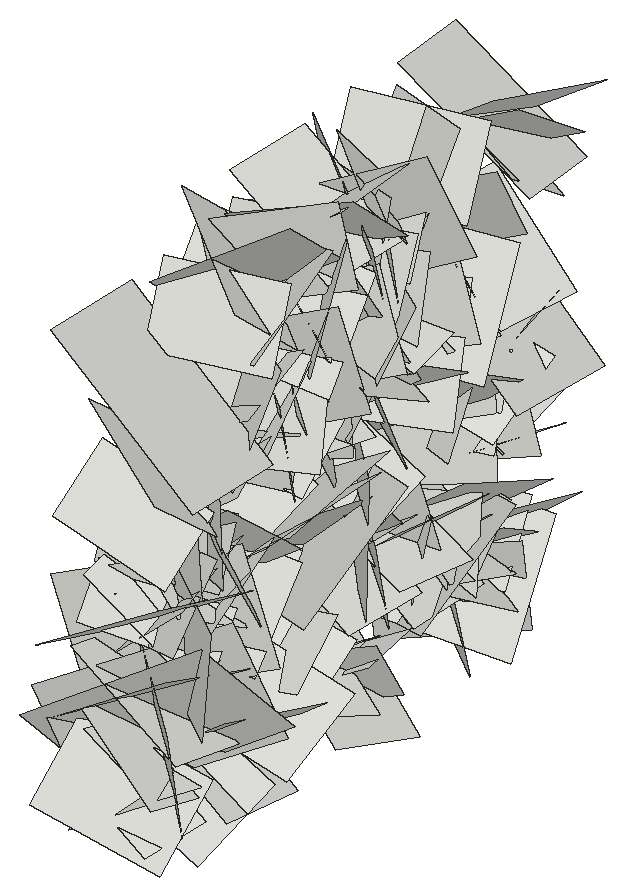
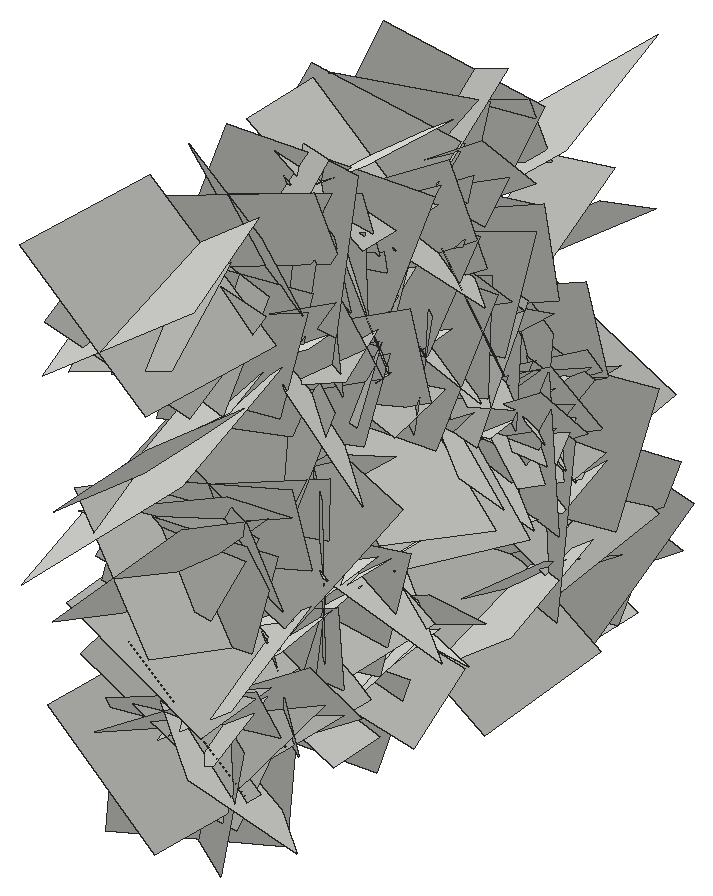
# SketchUp Ruby script. Lengths in inches.
U = 1.inch
M = Sketchup.active_model
def pt(a) = Geom::Point3d.new(a.map { |v| v * U })
def face(e, loops, mat)
  f = e.add_face(loops[0].map { |a| pt(a) })
  loops[1..].each { |l| e.add_face(l.map { |a| pt(a) }).erase! }
  f.material = f.back_material = mat if mat
  f
end
# faces: each face lists its corners as indices into pts; further lists are holes
def faces(e, pts, list, mat = nil) = list.each { |f| face(e, (f[0].is_a?(Array) ? f : [f]).map { |l| l.map { |i| pts[i] } }, mat) }
# xy, xz, yz: faces in a plane at the given z, y or x. An outline is a flat list of corners, or four numbers for a rectangle; further outlines are holes
def ring(l) = l.size == 4 ? [[l[0], l[1]], [l[2], l[1]], [l[2], l[3]], [l[0], l[3]]] : l.each_slice(2).to_a
def flat(e, list, mat, &to3) = list.each { |f| face(e, (f[0].is_a?(Array) ? f : [f]).map { |l| ring(l).map { |u, v| to3.(u, v) } }, mat) }
def xy(e, z, list, mat = nil) = flat(e, list, mat) { |x, y| [x, y, z] }
def xz(e, y, list, mat = nil) = flat(e, list, mat) { |x, z| [x, y, z] }
def yz(e, x, list, mat = nil) = flat(e, list, mat) { |y, z| [x, y, z] }
def lines(e, pts, list) = list.each { |a, b| e.add_line(pt(pts[a]), pt(pts[b])) }
# prism: a flat outline (further loops are holes) pulled along v
def prism(e, loops, v, mat = nil)
  f = face(e, loops, mat); d = Geom::Vector3d.new(v.map { |x| x * U })
  f.pushpull(f.normal.samedirection?(d) ? d.length : -d.length)
end
def box(e, o, s, mat = nil) = prism(e, [[o, [o[0] + s[0], o[1], o[2]], [o[0] + s[0], o[1] + s[1], o[2]], [o[0], o[1] + s[1], o[2]]]], [0, 0, s[2]], mat)
def at(x, y, z, deg = 0) = Geom::Transformation.translation(pt([x, y, z])) * Geom::Transformation.rotation(ORIGIN, Z_AXIS, deg.degrees)
def axes(o, x, y, z) = Geom::Transformation.new([*x, 0, *y, 0, *z, 0, *pt(o).to_a, 1])
def part(name) = M.definitions.add(name)
# library, detail: a bought-in or finely detailed component or shape, given as its bounding box
def library(name, o, s) = part(name).tap { |d| box(d.entities, o, s) }
def detail(e, o, s) = box(e.add_group.entities, o, s)
def put(e, d, t, mat = nil) = e.add_instance(d, t).tap { |i| i.material = mat if mat }
def group(e, t, mat = nil) = e.add_group.tap { |g| g.transformation = t; g.material = mat if mat }.entities
root = M.entities
c1 = part("Component\#6")
p = [[0.01,0,0],[0,3.24,4.54],[4.32,3.24,4.54],[4.33,0,0]]
faces(c1.entities,p,[[0,1,2,3]])
put(root,c1,axes([400.91,169.05,21.98],[0.04882,0.58162,0.59704],[-0.02934,0.59868,-0.58109],[0.88303,-0.01226,-0.05232]))
put(root,c1,axes([404.88,173.67,32.24],[0.05341,-0.65994,-0.37026],[0.06447,-0.36634,0.66124],[-0.79951,-0.07362,0.02859]))
put(root,c1,axes([404.88,173.11,21.9],[0.05319,-0.68826,0.19248],[0.04456,0.19546,0.68797],[-0.75624,-0.03689,0.05408]))
put(root,c1,axes([400.91,173.29,20.87],[0.09428,-0.62013,-0.08152],[0.03551,-0.0775,0.6261],[0.66205,0.09247,-0.02197]))
put(root,c1,axes([404.88,173.29,20.87],[-0.09428,-0.62013,-0.08152],[-0.03551,-0.0775,0.6261],[-0.66205,0.09247,-0.02197]))
put(root,c1,axes([404.88,173.15,22.23],[-0.01199,-0.5915,0.12784],[-0.10227,0.12799,0.58366],[-0.63327,-0.00947,-0.09668]))
put(root,c1,axes([400.91,174.01,26.46],[-0.07872,-0.97306,0.24072],[0.0738,0.23579,0.97461],[1.05998,-0.08868,-0.04998]))
put(root,c1,axes([400.91,172.13,35.78],[0.07615,0.65901,-0.5201],[0.04859,-0.52431,-0.658],[0.88857,-0.02781,0.08055]))
put(root,c1,axes([400.91,173.5,20.5],[-0.29119,-0.77592,0.90535],[0.00734,0.92801,0.79744],[1.26387,-0.18415,0.20396]))
put(root,c1,axes([404.88,171.18,26.98],[0.09963,0.88743,-0.23237],[-0.05305,-0.22828,-0.89204],[-0.97094,0.10354,0.02489]))
put(root,c1,axes([400.91,171.18,26.98],[-0.09963,0.88743,-0.23237],[0.05305,-0.22828,-0.89204],[0.97094,0.10354,0.02489]))
put(root,c1,axes([400.91,170.16,39.2],[-0.24703,1.2789,-0.21613],[-0.13589,-0.24123,-1.28918],[1.36812,0.20696,-0.16707]))
put(root,c1,axes([404.88,172,20.82],[0.19013,-0.4174,1.11707],[0.18593,1.12659,0.39279],[-1.25031,0.10406,0.22828]))
put(root,c1,axes([400.91,172,20.82],[-0.19013,-0.4174,1.11707],[-0.18593,1.12659,0.39279],[1.25031,0.10406,0.22828]))
put(root,c1,axes([400.91,171.52,27.71],[-0.03995,0.48298,0.66079],[-0.01207,0.66111,-0.48387],[0.8675,0.03144,0.0237]))
put(root,c1,axes([404.88,171.52,27.71],[0.03995,0.48298,0.66079],[0.01207,0.66111,-0.48387],[-0.8675,0.03144,0.0237]))
put(root,c1,axes([400.91,171.36,22.89],[0.02535,0.88672,0.32576],[-0.06435,0.32663,-0.88464],[0.99927,-0.00146,-0.06523]))
put(root,c1,axes([404.88,175.14,30.45],[0.22771,0.17317,-1.07869],[-0.0194,-1.09862,-0.18001],[-1.15789,0.05246,-0.20912]))
put(root,c1,axes([400.91,175.14,30.45],[-0.22771,0.17317,-1.07869],[0.0194,-1.09862,-0.18001],[1.15789,0.05246,-0.20912]))
put(root,c1,axes([404.88,174.95,31.63],[-0.12097,-0.07785,-0.70642],[-0.09105,-0.70871,0.09198],[-0.74781,0.09888,0.10307]))
put(root,c1,axes([400.91,174.95,31.63],[0.12097,-0.07785,-0.70642],[0.09105,-0.70871,0.09198],[0.74781,0.09888,0.10307]))
put(root,c1,axes([404.88,176.52,27.27],[-0.06139,-0.83333,-0.30669],[0.14477,-0.31205,0.82208],[-0.93005,0.00643,0.1482]))
put(root,c1,axes([400.91,176.52,27.27],[0.06139,-0.83333,-0.30669],[-0.14477,-0.31205,0.82208],[0.93005,0.00643,0.1482]))
put(root,c1,axes([404.88,174.16,29.86],[-0.19319,0.59277,-0.26834],[-0.07097,-0.29428,-0.60458],[-0.68606,-0.13648,0.1381]))
put(root,c1,axes([400.91,174.16,29.86],[0.19319,0.59277,-0.26834],[0.07097,-0.29428,-0.60458],[0.68606,-0.13648,0.1381]))
put(root,c1,axes([400.91,176.41,32.2],[0.11408,-0.0942,-0.79779],[0.0272,-0.8041,0.09841],[0.85109,0.03832,0.10379]))
put(root,c1,axes([400.91,172.625,27.43],[-0.01975,0.58315,0.74345],[0.01761,0.74368,-0.58292],[1.00141,-0.00157,0.02491]))
put(root,c1,axes([404.88,174.375,32.02],[0.18574,0.64681,-0.5499],[0.00393,-0.56207,-0.65994],[-0.8999,0.13105,-0.11638]))
put(root,c1,axes([400.91,176.05,33.17],[0.01986,0.50916,-0.88553],[-0.06176,-0.8837,-0.50934],[1.08099,-0.05984,-0.01283]))
put(root,c1,axes([404.88,178.05,19.9375],[0.14578,-1.0409,0.22357],[0.02192,0.228,1.04879],[-1.1283,-0.13006,0.04926]))
put(root,c1,axes([400.91,178.05,19.9375],[-0.14578,-1.0409,0.22357],[-0.02192,0.228,1.04879],[1.1283,-0.13006,0.04926]))
put(root,c1,axes([404.88,177.7,39.03],[0.08239,-0.33737,-0.64844],[-0.10668,-0.65083,0.32654],[-0.76743,0.05425,-0.11501]))
put(root,c1,axes([400.91,173.36,27.66],[-0.12062,0.63946,0.63128],[-0.06443,0.62939,-0.6485],[0.9503,0.12384,0.03616]))
put(root,c1,axes([404.88,173.36,27.66],[0.12062,0.63946,0.63128],[0.06443,0.62939,-0.6485],[-0.9503,0.12384,0.03616]))
put(root,c1,axes([404.88,174.875,32.24],[-0.12053,0.70886,0.38052],[0.08644,0.39248,-0.70676],[-0.84842,-0.06072,-0.12606]))
put(root,c1,axes([400.91,174.875,32.24],[0.12053,0.70886,0.38052],[-0.08644,0.39248,-0.70676],[0.84842,-0.06072,-0.12606]))
put(root,c1,axes([404.88,178.15,33.23],[-0.08938,-0.00525,-0.60269],[0.06829,-0.60515,-0.00374],[-0.63521,-0.06432,0.0844]))
put(root,c1,axes([404.88,174.67,32.54],[0.17055,0.3665,0.95024],[0.03456,0.95968,-0.37566],[-1.07902,0.08867,0.13816]))
put(root,c1,axes([400.91,174.67,32.54],[-0.17055,0.3665,0.95024],[-0.03456,0.95968,-0.37566],[1.07902,0.08867,0.13816]))
put(root,c1,axes([400.91,174.9,23.69],[-0.06803,0.90477,0.33383],[0.16872,0.33992,-0.89067],[1.00823,0.00417,0.17157]))
put(root,c1,axes([404.88,175.43,34.87],[0.0411,0.62613,0.35799],[0.03637,0.3565,-0.62724],[-0.76365,0.05068,-0.01061]))
put(root,c1,axes([404.88,178.01,36.42],[-0.04909,-0.68925,0.58112],[0.09024,0.57594,0.68989],[-0.95135,0.0902,0.03545]))
put(root,c1,axes([400.91,178.01,36.42],[0.04909,-0.68925,0.58112],[-0.09024,0.57594,0.68989],[0.95135,0.0902,0.03545]))
put(root,c1,axes([400.91,177.13,31.79],[-0.078,-0.30439,1.03044],[-0.07955,1.03178,0.29943],[1.13614,0.05135,0.09171]))
put(root,c1,axes([404.88,176.26,32.94],[-0.03084,0.60524,0.59943],[0.03406,0.60013,-0.60439],[-0.90231,0.00196,-0.0433]))
put(root,c1,axes([400.91,176.26,32.94],[0.03084,0.60524,0.59943],[-0.03406,0.60013,-0.60439],[0.90231,0.00196,-0.0433]))
put(root,c1,axes([400.91,182.1,27.04],[-0.18817,-1.1788,-0.21223],[-0.10509,-0.19936,1.19019],[1.26526,-0.19187,0.06729]))
put(root,c1,axes([400.91,175.72,36.8],[-0.15665,0.75943,0.7145],[-0.11122,0.70715,-0.77331],[1.09966,0.17971,0.02357]))
put(root,c1,axes([404.88,175.72,36.8],[0.15665,0.75943,0.7145],[0.11122,0.70715,-0.77331],[-1.09966,0.17971,0.02357]))
put(root,c1,axes([404.88,180.11,41],[0.0874,0.13713,-0.78202],[0.02965,-0.78624,-0.13492],[-0.84107,-0.01347,-0.08602]))
put(root,c1,axes([404.88,177.89,30.77],[-0.05678,-0.11721,0.8526],[0.09083,0.84928,0.12214],[-0.90772,0.09231,-0.04111]))
put(root,c1,axes([400.91,177.89,30.77],[0.05678,-0.11721,0.8526],[-0.09083,0.84928,0.12214],[0.90772,0.09231,-0.04111]))
put(root,c1,axes([404.88,177.99,23.55],[-0.04107,0.5427,0.4395],[-0.20397,0.41484,-0.52921],[-0.71159,-0.15024,0.12632]))
put(root,c1,axes([400.91,177.99,23.55],[0.04107,0.5427,0.4395],[0.20397,0.41484,-0.52921],[0.71159,-0.15024,0.12632]))
put(root,c1,axes([400.91,182.77,28.15],[-0.11013,-1.0722,-0.31704],[-0.03816,-0.31503,1.07721],[1.18456,-0.10983,0.00522]))
put(root,c1,axes([400.91,180.66,33.34],[-0.08177,-0.45253,0.73357],[0.03972,0.73405,0.45677],[0.91278,-0.07248,0.04584]))
put(root,c1,axes([404.88,180.66,33.34],[0.08177,-0.45253,0.73357],[-0.03972,0.73405,0.45677],[-0.91278,-0.07248,0.04584]))
put(root,c1,axes([404.88,182.27,37.76],[0.22679,0.05489,-0.89691],[0.06736,-0.9206,-0.04118],[-0.95012,-0.05216,-0.217]))
put(root,c1,axes([404.88,182.09,31.375],[-0.0562,-0.72005,0.10613],[-0.07977,0.11126,0.71729],[-0.76737,0.04117,-0.08234]))
put(root,c1,axes([400.91,182.09,31.375],[0.0562,-0.72005,0.10613],[0.07977,0.11126,0.71729],[0.76737,0.04117,-0.08234]))
put(root,c1,axes([404.88,180.04,24.28],[-0.15161,0.71603,-0.23582],[-0.04269,-0.24694,-0.72538],[-0.79796,-0.12284,0.08362]))
put(root,c1,axes([400.91,180.04,24.28],[0.15161,0.71603,-0.23582],[0.04269,-0.24694,-0.72538],[0.79796,-0.12284,0.08362]))
put(root,c1,axes([400.91,181.67,36.78],[-0.05967,0.56874,-0.94691],[-0.29528,-0.9248,-0.5389],[1.13301,-0.21107,-0.19031]))
put(root,c1,axes([404.88,181.67,36.78],[0.05967,0.56874,-0.94691],[0.29528,-0.9248,-0.5389],[-1.13301,-0.21107,-0.19031]))
put(root,c1,axes([400.91,181.8125,37.17],[-0.0246,-0.63961,0.56311],[0.17949,0.54862,0.63013],[0.88529,-0.129,-0.11211]))
put(root,c1,axes([404.88,184.3,37.98],[0.01849,-0.42221,-1.00939],[0.24573,-0.98518,0.41609],[-1.13346,-0.22047,0.07374]))
put(root,c1,axes([400.91,184.3,37.98],[-0.01849,-0.42221,-1.00939],[-0.24573,-0.98518,0.41609],[1.13346,-0.22047,0.07374]))
put(root,c1,axes([400.91,185.38,28.27],[-0.28552,-0.8956,-0.93898],[-0.07116,-0.9481,0.92355],[1.37362,-0.23528,-0.14733]))
put(root,c1,axes([404.88,183.5625,38.07],[-0.03427,-0.86867,-0.02883],[0.01016,-0.0292,0.8692],[-0.92124,0.03199,0.01066]))
put(root,c1,axes([400.91,183.5625,38.07],[0.03427,-0.86867,-0.02883],[-0.01016,-0.0292,0.8692],[0.92124,0.03199,0.01066]))
put(root,c1,axes([404.88,181.88,29.24],[-0.0732,0.47057,-0.46808],[0.06498,-0.46407,-0.47558],[-0.70054,-0.09222,0.00479]))
put(root,c1,axes([400.91,180.55,24.45],[0.04702,0.95483,-0.28451],[-0.08229,-0.28062,-0.95386],[1.05288,-0.06457,-0.06184]))
put(root,c1,axes([404.88,182.11,23.57],[0.01533,0.32032,-0.55846],[-0.07998,-0.55391,-0.31966],[-0.67773,0.07262,0.02509]))
put(root,c1,axes([404.88,180.54,27.52],[-0.00647,0.86334,-0.00303],[0.00368,-0.003,-0.86336],[-0.91514,-0.00612,-0.00345]))
put(root,c1,axes([400.91,180.54,27.52],[0.00647,0.86334,-0.00303],[-0.00368,-0.003,-0.86336],[0.91514,-0.00612,-0.00345]))
put(root,c1,axes([400.91,181.12,36.49],[-0.0887,0.85058,-0.45713],[0.14057,-0.44437,-0.85112],[1.01388,0.13603,0.07801]))
put(root,c1,axes([404.88,184.65,28.76],[-0.04824,-0.62434,-0.28052],[0.09786,-0.28417,0.61748],[-0.7189,0.00321,0.10288]))
put(root,c1,axes([400.91,185.4,30.76],[-0.02152,-0.00963,-1.2106],[-0.23963,-1.18945,0.01326],[1.26071,-0.22625,-0.01814]))
put(root,c1,axes([404.88,181.75,22.9],[-0.07496,0.59984,0.04506],[-0.05269,0.03939,-0.60235],[-0.63545,-0.07402,0.04463]))
put(root,c1,axes([400.91,184.92,37.05],[0.01613,-0.13323,-0.78421],[0.01491,-0.78419,0.1335],[0.84304,0.01642,0.01265]))
put(root,c1,axes([404.88,184.92,37.05],[-0.01613,-0.13323,-0.78421],[-0.01491,-0.78419,0.1335],[-0.84304,0.01642,0.01265]))
put(root,c1,axes([404.88,182.91,34.72],[0.14912,-0.41506,0.98502],[0.044,0.99488,0.41329],[-1.13217,-0.016,0.1458]))
put(root,c1,axes([400.91,182.91,34.72],[-0.14912,-0.41506,0.98502],[-0.044,0.99488,0.41329],[1.13217,-0.016,0.1458]))
put(root,c1,axes([400.91,184.84,39.1],[0.02023,-0.20369,-0.6632],[0.11732,-0.65406,0.20407],[0.72599,0.11137,-0.0145]))
put(root,c1,axes([404.88,184.84,39.1],[-0.02023,-0.20369,-0.6632],[-0.11732,-0.65406,0.20407],[-0.72599,0.11137,-0.0145]))
put(root,c1,axes([400.91,182.78,23.92],[-0.06221,-0.24398,0.83625],[-0.07047,0.83695,0.23952],[0.92069,0.04758,0.07484]))
put(root,c1,axes([404.88,182.78,23.92],[0.06221,-0.24398,0.83625],[0.07047,0.83695,0.23952],[-0.92069,0.04758,0.07484]))
put(root,c1,axes([400.91,184.8,33.37],[0.19651,0.19461,-0.78555],[-0.01158,-0.80522,-0.20206],[0.85778,-0.05545,0.17724]))
put(root,c1,axes([404.88,187.08,35.11],[0.23629,-0.52338,-1.02054],[0.13084,-1.02265,0.55142],[-1.20867,-0.21302,-0.13982]))
put(root,c1,axes([400.91,187.08,35.11],[-0.23629,-0.52338,-1.02054],[-0.13084,-1.02265,0.55142],[1.20867,-0.21302,-0.13982]))
put(root,c1,axes([404.88,183.74,37.84],[-0.08456,-0.37494,0.46177],[0.03825,0.46199,0.38136],[-0.62935,0.07846,-0.03886]))
put(root,c1,axes([400.91,183.3,35.54],[0.06853,-0.0517,0.64839],[0.02911,0.65122,0.04919],[0.68886,-0.02238,-0.06659]))
put(root,c1,axes([404.88,183.3,35.54],[-0.06853,-0.0517,0.64839],[-0.02911,0.65122,0.04919],[-0.68886,-0.02238,-0.06659]))
put(root,c1,axes([404.88,186.27,36.66],[0.23271,0.08267,-1.0169],[0.17131,-1.02986,-0.04883],[-1.06781,-0.14721,-0.22945]))
put(root,c1,axes([400.91,182.86,27.86],[0.00866,0.87216,-0.09866],[0.12421,-0.09886,-0.86427],[0.92206,0.00513,0.11735]))
put(root,c1,axes([404.88,186.9,33.68],[0.12726,-0.80704,-0.07778],[-0.05104,-0.08559,0.81372],[-0.85791,-0.11462,-0.05995]))
put(root,c1,axes([400.91,186.8,27.07],[-0.11611,-1.02809,0.5245],[-0.14127,0.5346,1.02006],[1.21522,-0.03608,0.16869]))
put(root,c1,axes([400.91,187.74,23.43],[-0.08523,-0.9506,0.05636],[-0.09187,0.06363,0.94959],[1.00521,-0.07479,0.09156]))
put(root,c1,axes([404.88,187.74,23.43],[0.08523,-0.9506,0.05636],[0.09187,0.06363,0.94959],[-1.00521,-0.07479,0.09156]))
put(root,c1,axes([400.91,182.62,33.52],[-0.16113,0.63843,0.91206],[-0.00988,0.91976,-0.64538],[1.18006,0.09488,0.11913]))
put(root,c1,axes([400.91,187.61,26.86],[-0.07932,-0.16974,-0.83453],[-0.0041,-0.83766,0.17072],[0.9027,-0.01872,-0.07255]))
put(root,c1,axes([404.88,187.61,26.86],[0.07932,-0.16974,-0.83453],[0.0041,-0.83766,0.17072],[-0.9027,-0.01872,-0.07255]))
put(root,c1,axes([404.88,188.3,31.13],[0.1103,-0.11339,-0.88165],[0.13763,-0.87621,0.12802],[-0.93214,-0.14279,-0.08543]))
put(root,c1,axes([400.91,184.52,38.07],[-0.06477,0.36641,0.7198],[0.11209,0.71927,-0.35717],[0.84878,-0.06703,0.10209]))
put(root,c1,axes([404.88,184.52,38.07],[0.06477,0.36641,0.7198],[-0.11209,0.71927,-0.35717],[-0.84878,-0.06703,0.10209]))
put(root,c1,axes([404.88,188.62,32.29],[0.0866,-0.74743,0.19758],[0.06186,0.20408,0.74787],[-0.81715,-0.06376,0.07755]))
put(root,c1,axes([404.88,185.86,28.71],[0.06844,0.29244,0.76285],[-0.17475,0.75415,-0.27515],[-0.84819,-0.13178,0.11824]))
put(root,c1,axes([400.91,185.86,28.71],[-0.06844,0.29244,0.76285],[0.17475,0.75415,-0.27515],[0.84819,-0.13178,0.11824]))
put(root,c1,axes([404.88,187.32,34.27],[-0.05201,-0.4187,0.7383],[0.02779,0.73844,0.42051],[-0.89926,0.04704,-0.0297]))
put(root,c1,axes([400.91,187.32,34.27],[0.05201,-0.4187,0.7383],[-0.02779,0.73844,0.42051],[0.89926,0.04704,-0.0297]))
put(root,c1,axes([404.88,191.48,24.4],[0.24044,-0.84726,-0.84182],[0.11443,-0.83882,0.87332],[-1.26085,-0.2377,-0.08127]))
put(root,c1,axes([400.91,191.48,24.4],[-0.24044,-0.84726,-0.84182],[-0.11443,-0.83882,0.87332],[1.26085,-0.2377,-0.08127]))
put(root,c1,axes([400.91,186.85,26],[0.04759,0.74401,-0.43208],[0.09551,-0.43435,-0.73856],[0.90698,0.0067,0.10045]))
put(root,c1,axes([404.88,189.58,22.99],[0.08755,-0.94666,0.34405],[0.04779,0.34833,0.94763],[-1.06661,-0.0621,0.0707]))
put(root,c1,axes([400.91,189.58,22.99],[-0.08755,-0.94666,0.34405],[-0.04779,0.34833,0.94763],[1.06661,-0.0621,0.0707]))
put(root,c1,axes([404.88,186.99,20.26],[-0.04681,-0.17583,0.86867],[0.05724,0.86759,0.17835],[-0.93771,0.06173,-0.03248]))
put(root,c1,axes([400.91,186.99,20.26],[0.04681,-0.17583,0.86867],[-0.05724,0.86759,0.17835],[0.93771,0.06173,-0.03248]))
put(root,c1,axes([400.91,186.48,30.64],[0.03295,0.70699,0.47041],[0.18441,0.45544,-0.69599],[0.88105,-0.12176,0.12808]))
put(root,c1,axes([404.88,189.49,31],[0.19159,0.03614,-0.77666],[-0.1449,-0.78347,-0.06827],[-0.81131,0.14846,-0.17121]))
put(root,c1,axes([400.91,189.24,21.76],[0.15995,-0.688,0.38857],[-0.02017,0.39231,0.70202],[0.83731,0.14088,-0.05731]))
put(root,c1,axes([400.91,186.98,23.44],[-0.07046,0.41434,0.63319],[0.10971,0.63463,-0.40442],[0.79457,-0.05088,0.11199]))
put(root,c1,axes([404.88,186.98,23.44],[0.07046,0.41434,0.63319],[-0.10971,0.63463,-0.40442],[-0.79457,-0.05088,0.11199]))
put(root,c1,axes([400.91,190.89,25.45],[-0.07637,-0.93381,0.1535],[0.06656,0.14888,0.93522],[1.00091,-0.08115,-0.05048]))
put(root,c1,axes([404.88,188.48,31.6],[-0.00806,0.51701,-0.38199],[-0.06142,-0.38101,-0.51453],[-0.67861,0.02834,0.0511]))
put(root,c1,axes([400.91,187.18,35.87],[-0.21905,1.32848,-0.23139],[-0.18572,-0.25856,-1.32798],[1.41727,0.17144,-0.20979]))
put(root,c1,axes([404.88,188.01,25.87],[0.18323,0.88768,-0.1275],[0.06793,-0.14175,-0.89995],[-0.94816,0.16139,-0.08912]))
put(root,c1,axes([400.91,187.84,31.26],[0.01205,0.8882,0.30464],[-0.22592,0.29915,-0.86424],[0.96935,0.05868,-0.20521]))
put(root,c1,axes([404.88,187.84,31.26],[-0.01205,0.8882,0.30464],[0.22592,0.29915,-0.86424],[-0.96935,0.05868,-0.20521]))
put(root,c1,axes([404.88,189.53,40.3125],[0.07096,0.70634,-0.4758],[-0.12627,-0.46481,-0.70678],[-0.89387,0.12173,0.06207]))
put(root,c1,axes([400.91,189.53,40.3125],[-0.07096,0.70634,-0.4758],[0.12627,-0.46481,-0.70678],[0.89387,0.12173,0.06207]))
put(root,c1,axes([400.91,188.23,41.22],[-0.26749,1.02168,-0.17372],[0.00845,-0.17688,-1.05183],[1.0985,0.25014,-0.03421]))
put(root,c1,axes([404.88,188.23,41.22],[0.26749,1.02168,-0.17372],[-0.00845,-0.17688,-1.05183],[-1.0985,0.25014,-0.03421]))
put(root,c1,axes([404.88,192.58,32.17],[-0.11188,-0.86522,-0.03173],[0.14554,-0.04829,0.85998],[-0.90613,0.09907,0.14204]))
